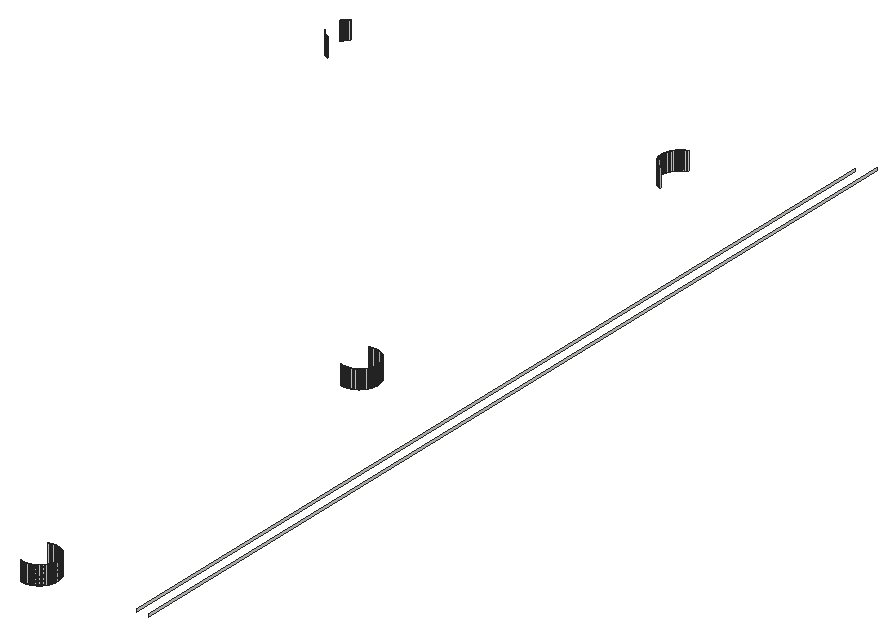
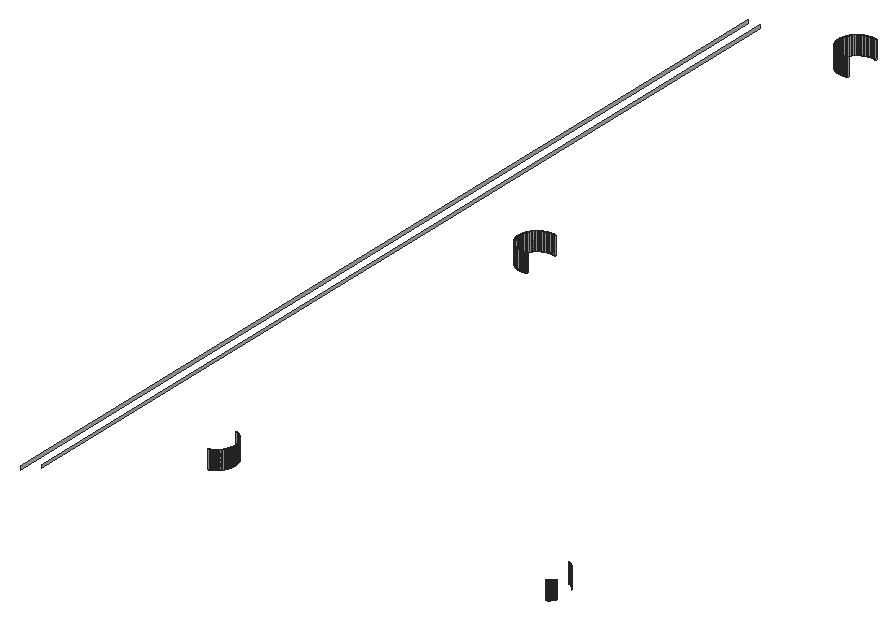
# SketchUp Ruby script. Lengths in inches.
U = 1.inch
M = Sketchup.active_model
def pt(a) = Geom::Point3d.new(a.map { |v| v * U })
def face(e, loops, mat)
  f = e.add_face(loops[0].map { |a| pt(a) })
  loops[1..].each { |l| e.add_face(l.map { |a| pt(a) }).erase! }
  f.material = f.back_material = mat if mat
  f
end
# faces: each face lists its corners as indices into pts; further lists are holes
def faces(e, pts, list, mat = nil) = list.each { |f| face(e, (f[0].is_a?(Array) ? f : [f]).map { |l| l.map { |i| pts[i] } }, mat) }
# xy, xz, yz: faces in a plane at the given z, y or x. An outline is a flat list of corners, or four numbers for a rectangle; further outlines are holes
def ring(l) = l.size == 4 ? [[l[0], l[1]], [l[2], l[1]], [l[2], l[3]], [l[0], l[3]]] : l.each_slice(2).to_a
def flat(e, list, mat, &to3) = list.each { |f| face(e, (f[0].is_a?(Array) ? f : [f]).map { |l| ring(l).map { |u, v| to3.(u, v) } }, mat) }
def xy(e, z, list, mat = nil) = flat(e, list, mat) { |x, y| [x, y, z] }
def xz(e, y, list, mat = nil) = flat(e, list, mat) { |x, z| [x, y, z] }
def yz(e, x, list, mat = nil) = flat(e, list, mat) { |y, z| [x, y, z] }
def lines(e, pts, list) = list.each { |a, b| e.add_line(pt(pts[a]), pt(pts[b])) }
# prism: a flat outline (further loops are holes) pulled along v
def prism(e, loops, v, mat = nil)
  f = face(e, loops, mat); d = Geom::Vector3d.new(v.map { |x| x * U })
  f.pushpull(f.normal.samedirection?(d) ? d.length : -d.length)
end
def box(e, o, s, mat = nil) = prism(e, [[o, [o[0] + s[0], o[1], o[2]], [o[0] + s[0], o[1] + s[1], o[2]], [o[0], o[1] + s[1], o[2]]]], [0, 0, s[2]], mat)
def at(x, y, z, deg = 0) = Geom::Transformation.translation(pt([x, y, z])) * Geom::Transformation.rotation(ORIGIN, Z_AXIS, deg.degrees)
def axes(o, x, y, z) = Geom::Transformation.new([*x, 0, *y, 0, *z, 0, *pt(o).to_a, 1])
def part(name) = M.definitions.add(name)
# library, detail: a bought-in or finely detailed component or shape, given as its bounding box
def library(name, o, s) = part(name).tap { |d| box(d.entities, o, s) }
def detail(e, o, s) = box(e.add_group.entities, o, s)
def put(e, d, t, mat = nil) = e.add_instance(d, t).tap { |i| i.material = mat if mat }
def group(e, t, mat = nil) = e.add_group.tap { |g| g.transformation = t; g.material = mat if mat }.entities
root = M.entities
xz(root,185,[[323.875,231,323.95,234],[323.95,231,324.03,234],[324.03,231,324.11,234]])
xz(root,185.01,[[323.72,231,323.8,234],[324.19,231,324.27,234]])
xz(root,190.99,[[323.73,231,323.81,234],[324.2,231,324.28,234]])
xz(root,191,[[323.89,231,323.97,234],[323.97,231,324.05,234],[324.05,231,324.125,234]])
xz(root,251,[[323.875,231,323.95,234],[323.95,231,324.03,234],[324.03,231,324.11,234]])
xz(root,251.01,[[323.72,231,323.8,234],[324.19,231,324.27,234]])
xz(root,256.99,[[323.73,231,323.81,234],[324.2,231,324.28,234]])
xz(root,257,[[323.89,231,323.97,234],[323.97,231,324.05,234],[324.05,231,324.125,234]])
yz(root,321,[[319.89,231,319.97,234],[319.97,231,320.05,234],[320.05,231,320.125,234]])
yz(root,321.01,[[319.73,231,319.81,234],[320.2,231,320.28,234]])
yz(root,326.99,[[187.72,231,187.8,234],[188.19,231,188.27,234],[253.72,231,253.8,234],[254.19,231,254.27,234]])
yz(root,327,[[187.875,231,187.95,234],[187.95,231,188.03,234],[188.03,231,188.11,234],[253.875,231,253.95,234],[253.95,231,254.03,234],
  [254.03,231,254.11,234]])
yz(root,340,[[188,231,336,231.5]])
yz(root,342,[[188,231,338,231.5]])
p = [[323.49,185.04,231],[323.41,185.06,231],[323.41,185.06,234],[323.49,185.04,234],[323.5625,185.03,231],[323.5625,185.03,234],
  [323.64,185.02,231],[323.64,185.02,234],[323.72,185.01,231],[323.72,185.01,234],[323.875,185,231],[323.8,185.01,231],
  [323.8,185.01,234],[323.875,185,234],[324.19,185.01,231],[324.11,185,231],[324.11,185,234],[324.19,185.01,234],
  [324.35,185.02,231],[324.27,185.01,231],[324.27,185.01,234],[324.35,185.02,234],[324.42,185.03,231],[324.42,185.03,234],
  [324.5,185.04,231],[324.5,185.04,234],[324.58,185.06,231],[324.58,185.06,234],[323.18,185.11,231],[323.1,185.14,231],
  [323.1,185.14,234],[323.18,185.11,234],[323.26,185.09,231],[323.26,185.09,234],[323.33,185.08,231],[323.33,185.08,234],
  [324.66,185.07,231],[324.66,185.07,234],[324.73,185.09,231],[324.73,185.09,234],[324.81,185.11,231],[324.81,185.11,234],
  [324.88,185.13,231],[324.88,185.13,234],[324.96,185.16,231],[324.96,185.16,234],[325.03,185.18,231],[325.03,185.18,234],
  [325.11,185.21,231],[325.11,185.21,234],[325.18,185.24,231],[325.18,185.24,234],[325.25,185.27,231],[325.25,185.27,234],
  [325.32,185.31,231],[325.32,185.31,234],[325.39,185.34,231],[325.39,185.34,234],[325.46,185.38,231],[325.46,185.38,234],
  [325.53,185.42,231],[325.53,185.42,234],[325.6,185.46,231],[325.6,185.46,234],[325.66,185.5,231],[325.66,185.5,234],
  [325.73,185.55,231],[325.73,185.55,234],[325.79,185.59,231],[325.79,185.59,234],[325.85,185.64,231],[325.85,185.64,234],
  [325.91,185.69,231],[325.91,185.69,234],[325.97,185.74,231],[325.97,185.74,234],[326.03,185.79,231],[326.03,185.79,234],
  [326.09,185.85,231],[326.09,185.85,234],[326.14,185.9,231],[326.14,185.9,234],[326.2,185.96,231],[326.2,185.96,234],
  [326.25,186.02,231],[326.25,186.02,234],[326.3,186.08,231],[326.3,186.08,234],[326.35,186.14,231],[326.35,186.14,234],
  [326.4,186.2,231],[326.4,186.2,234],[326.45,186.26,231],[326.45,186.26,234],[326.49,186.33,231],[326.49,186.33,234],
  [326.53,186.39,231],[326.53,186.39,234],[326.58,186.46,231],[326.58,186.46,234],[326.61,186.53,231],[326.61,186.53,234],
  [326.65,186.6,231],[326.65,186.6,234],[326.6875,186.67,231],[326.6875,186.67,234],[326.72,186.74,231],[326.72,186.74,234],
  [326.75,186.81,231],[326.75,186.81,234],[326.78,186.88,231],[326.78,186.88,234],[326.8125,186.96,231],[326.8125,186.96,234],
  [326.84,187.03,231],[326.84,187.03,234],[326.86,187.1,231],[326.86,187.1,234],[326.89,187.18,231],[326.89,187.18,234],
  [326.91,187.26,231],[326.91,187.26,234],[326.92,187.33,231],[326.92,187.33,234],[326.94,187.41,231],[326.94,187.41,234],
  [326.96,187.49,231],[326.96,187.49,234],[326.97,187.5625,231],[326.97,187.5625,234],[326.98,187.64,231],[326.98,187.64,234],
  [326.99,187.72,231],[326.99,187.72,234],[327,187.875,231],[326.99,187.8,231],[326.99,187.8,234],[327,187.875,234],
  [326.99,188.19,231],[327,188.11,231],[327,188.11,234],[326.99,188.19,234],[326.97,188.42,231],[326.98,188.35,231],
  [326.98,188.35,234],[326.97,188.42,234],[326.99,188.27,231],[326.99,188.27,234],[326.96,188.5,231],[326.96,188.5,234],
  [326.94,188.58,231],[326.94,188.58,234],[326.93,188.66,231],[326.93,188.66,234],[326.89,188.81,231],[326.91,188.73,231],
  [326.91,188.73,234],[326.89,188.81,234],[326.87,188.88,231],[326.87,188.88,234],[326.84,188.96,231],[326.84,188.96,234],
  [326.79,189.11,231],[326.82,189.03,231],[326.82,189.03,234],[326.79,189.11,234],[326.76,189.18,231],[326.76,189.18,234],
  [326.73,189.25,231],[326.73,189.25,234],[326.66,189.39,231],[326.69,189.32,231],[326.69,189.32,234],[326.66,189.39,234],
  [326.62,189.46,231],[326.62,189.46,234],[326.54,189.6,231],[326.58,189.53,231],[326.58,189.53,234],[326.54,189.6,234],
  [326.5,189.66,231],[326.5,189.66,234],[326.41,189.79,231],[326.45,189.73,231],[326.45,189.73,234],[326.41,189.79,234],
  [326.36,189.85,231],[326.36,189.85,234],[326.26,189.97,231],[326.31,189.91,231],[326.31,189.91,234],[326.26,189.97,234],
  [326.15,190.09,231],[326.21,190.03,231],[326.21,190.03,234],[326.15,190.09,234],[326.04,190.2,231],[326.1,190.14,231],
  [326.1,190.14,234],[326.04,190.2,234],[325.98,190.25,231],[325.98,190.25,234],[325.86,190.35,231],[325.92,190.3,231],
  [325.92,190.3,234],[325.86,190.35,234],[325.67,190.49,231],[325.74,190.45,231],[325.74,190.45,234],[325.67,190.49,234],
  [325.8,190.4,231],[325.8,190.4,234],[325.54,190.58,231],[325.61,190.53,231],[325.61,190.53,234],[325.54,190.58,234],
  [325.4,190.65,231],[325.47,190.61,231],[325.47,190.61,234],[325.4,190.65,234],[325.19,190.75,231],[325.26,190.72,231],
  [325.26,190.72,234],[325.19,190.75,234],[325.33,190.6875,231],[325.33,190.6875,234],[324.9,190.86,231],[324.97,190.84,231],
  [324.97,190.84,234],[324.9,190.86,234],[325.04,190.8125,231],[325.04,190.8125,234],[325.12,190.78,231],[325.12,190.78,234],
  [323.12,190.87,231],[323.19,190.89,231],[323.19,190.89,234],[323.12,190.87,234],[323.27,190.91,231],[323.27,190.91,234],
  [323.34,190.93,231],[323.34,190.93,234],[323.42,190.94,231],[323.42,190.94,234],[323.5,190.96,231],[323.5,190.96,234],
  [324.51,190.96,231],[324.59,190.94,231],[324.59,190.94,234],[324.51,190.96,234],[324.67,190.92,231],[324.67,190.92,234],
  [324.74,190.91,231],[324.74,190.91,234],[324.82,190.89,231],[324.82,190.89,234],[323.58,190.97,231],[323.58,190.97,234],
  [323.65,190.98,231],[323.65,190.98,234],[323.73,190.99,231],[323.73,190.99,234],[323.81,190.99,231],[323.89,191,231],
  [323.89,191,234],[323.81,190.99,234],[324.125,191,231],[324.2,190.99,231],[324.2,190.99,234],[324.125,191,234],
  [324.28,190.99,231],[324.36,190.98,231],[324.36,190.98,234],[324.28,190.99,234],[324.4375,190.97,231],[324.4375,190.97,234],
  [323.49,251.04,231],[323.41,251.06,231],[323.41,251.06,234],[323.49,251.04,234],[323.5625,251.03,231],[323.5625,251.03,234],
  [323.64,251.02,231],[323.64,251.02,234],[323.72,251.01,231],[323.72,251.01,234],[323.875,251,231],[323.8,251.01,231],
  [323.8,251.01,234],[323.875,251,234],[324.19,251.01,231],[324.11,251,231],[324.11,251,234],[324.19,251.01,234],
  [324.35,251.02,231],[324.27,251.01,231],[324.27,251.01,234],[324.35,251.02,234],[324.42,251.03,231],[324.42,251.03,234],
  [324.5,251.04,231],[324.5,251.04,234],[324.58,251.06,231],[324.58,251.06,234],[323.18,251.11,231],[323.1,251.14,231],
  [323.1,251.14,234],[323.18,251.11,234],[323.26,251.09,231],[323.26,251.09,234],[323.33,251.08,231],[323.33,251.08,234],
  [324.66,251.07,231],[324.66,251.07,234],[324.73,251.09,231],[324.73,251.09,234],[324.81,251.11,231],[324.81,251.11,234],
  [324.88,251.13,231],[324.88,251.13,234],[324.96,251.16,231],[324.96,251.16,234],[325.03,251.18,231],[325.03,251.18,234],
  [325.11,251.21,231],[325.11,251.21,234],[325.18,251.24,231],[325.18,251.24,234],[325.25,251.27,231],[325.25,251.27,234],
  [325.32,251.31,231],[325.32,251.31,234],[325.39,251.34,231],[325.39,251.34,234],[325.46,251.38,231],[325.46,251.38,234],
  [325.53,251.42,231],[325.53,251.42,234],[325.6,251.46,231],[325.6,251.46,234],[325.66,251.5,231],[325.66,251.5,234],
  [325.73,251.55,231],[325.73,251.55,234],[325.79,251.59,231],[325.79,251.59,234],[325.85,251.64,231],[325.85,251.64,234],
  [325.91,251.69,231],[325.91,251.69,234],[325.97,251.74,231],[325.97,251.74,234],[326.03,251.79,231],[326.03,251.79,234],
  [326.09,251.85,231],[326.09,251.85,234],[326.14,251.9,231],[326.14,251.9,234],[326.2,251.96,231],[326.2,251.96,234],
  [326.25,252.02,231],[326.25,252.02,234],[326.3,252.08,231],[326.3,252.08,234],[326.35,252.14,231],[326.35,252.14,234],
  [326.4,252.2,231],[326.4,252.2,234],[326.45,252.26,231],[326.45,252.26,234],[326.49,252.33,231],[326.49,252.33,234],
  [326.53,252.39,231],[326.53,252.39,234],[326.58,252.46,231],[326.58,252.46,234],[326.61,252.53,231],[326.61,252.53,234],
  [326.65,252.6,231],[326.65,252.6,234],[326.6875,252.67,231],[326.6875,252.67,234],[326.72,252.74,231],[326.72,252.74,234],
  [326.75,252.81,231],[326.75,252.81,234],[326.78,252.88,231],[326.78,252.88,234],[326.8125,252.96,231],[326.8125,252.96,234],
  [326.84,253.03,231],[326.84,253.03,234],[326.86,253.1,231],[326.86,253.1,234],[326.89,253.18,231],[326.89,253.18,234],
  [326.91,253.26,231],[326.91,253.26,234],[326.92,253.33,231],[326.92,253.33,234],[326.94,253.41,231],[326.94,253.41,234],
  [326.96,253.49,231],[326.96,253.49,234],[326.97,253.5625,231],[326.97,253.5625,234],[326.98,253.64,231],[326.98,253.64,234],
  [326.99,253.72,231],[326.99,253.72,234],[327,253.875,231],[326.99,253.8,231],[326.99,253.8,234],[327,253.875,234],
  [326.99,254.19,231],[327,254.11,231],[327,254.11,234],[326.99,254.19,234],[326.97,254.42,231],[326.98,254.35,231],
  [326.98,254.35,234],[326.97,254.42,234],[326.99,254.27,231],[326.99,254.27,234],[326.96,254.5,231],[326.96,254.5,234],
  [326.94,254.58,231],[326.94,254.58,234],[326.93,254.66,231],[326.93,254.66,234],[326.89,254.81,231],[326.91,254.73,231],
  [326.91,254.73,234],[326.89,254.81,234],[326.87,254.88,231],[326.87,254.88,234],[326.84,254.96,231],[326.84,254.96,234],
  [326.79,255.11,231],[326.82,255.03,231],[326.82,255.03,234],[326.79,255.11,234],[326.76,255.18,231],[326.76,255.18,234],
  [326.73,255.25,231],[326.73,255.25,234],[326.66,255.39,231],[326.69,255.32,231],[326.69,255.32,234],[326.66,255.39,234],
  [326.62,255.46,231],[326.62,255.46,234],[326.54,255.6,231],[326.58,255.53,231],[326.58,255.53,234],[326.54,255.6,234],
  [326.5,255.66,231],[326.5,255.66,234],[326.41,255.79,231],[326.45,255.73,231],[326.45,255.73,234],[326.41,255.79,234],
  [326.36,255.85,231],[326.36,255.85,234],[326.26,255.97,231],[326.31,255.91,231],[326.31,255.91,234],[326.26,255.97,234],
  [326.15,256.09,231],[326.21,256.03,231],[326.21,256.03,234],[326.15,256.09,234],[326.04,256.2,231],[326.1,256.14,231],
  [326.1,256.14,234],[326.04,256.2,234],[325.98,256.25,231],[325.98,256.25,234],[325.86,256.35,231],[325.92,256.3,231],
  [325.92,256.3,234],[325.86,256.35,234],[325.67,256.49,231],[325.74,256.45,231],[325.74,256.45,234],[325.67,256.49,234],
  [325.8,256.4,231],[325.8,256.4,234],[325.54,256.58,231],[325.61,256.53,231],[325.61,256.53,234],[325.54,256.58,234],
  [325.4,256.65,231],[325.47,256.61,231],[325.47,256.61,234],[325.4,256.65,234],[325.19,256.75,231],[325.26,256.72,231],
  [325.26,256.72,234],[325.19,256.75,234],[325.33,256.6875,231],[325.33,256.6875,234],[324.9,256.86,231],[324.97,256.84,231],
  [324.97,256.84,234],[324.9,256.86,234],[325.04,256.8125,231],[325.04,256.8125,234],[325.12,256.78,231],[325.12,256.78,234],
  [323.12,256.87,231],[323.19,256.89,231],[323.19,256.89,234],[323.12,256.87,234],[323.27,256.91,231],[323.27,256.91,234],
  [323.34,256.93,231],[323.34,256.93,234],[323.42,256.94,231],[323.42,256.94,234],[323.5,256.96,231],[323.5,256.96,234],
  [324.51,256.96,231],[324.59,256.94,231],[324.59,256.94,234],[324.51,256.96,234],[324.67,256.92,231],[324.67,256.92,234],
  [324.74,256.91,231],[324.74,256.91,234],[324.82,256.89,231],[324.82,256.89,234],[323.58,256.97,231],[323.58,256.97,234],
  [323.65,256.98,231],[323.65,256.98,234],[323.73,256.99,231],[323.73,256.99,234],[323.81,256.99,231],[323.89,257,231],
  [323.89,257,234],[323.81,256.99,234],[324.125,257,231],[324.2,256.99,231],[324.2,256.99,234],[324.125,257,234],
  [324.28,256.99,231],[324.36,256.98,231],[324.36,256.98,234],[324.28,256.99,234],[324.4375,256.97,231],[324.4375,256.97,234],
  [268.3,317.14,231],[268.23,317.16,231],[268.23,317.16,234],[268.3,317.14,234],[323.1,317.14,231],[323.03,317.16,231],
  [323.03,317.16,234],[323.1,317.14,234],[268.01,317.25,231],[267.9375,317.28,231],[267.9375,317.28,234],[268.01,317.25,234],
  [268.08,317.22,231],[268.08,317.22,234],[268.16,317.1875,231],[268.16,317.1875,234],[322.81,317.25,231],[322.74,317.28,231],
  [322.74,317.28,234],[322.81,317.25,234],[322.88,317.22,231],[322.88,317.22,234],[322.96,317.1875,231],[322.96,317.1875,234],
  [267.8,317.35,231],[267.73,317.39,231],[267.73,317.39,234],[267.8,317.35,234],[267.87,317.3125,231],[267.87,317.3125,234],
  [322.6,317.35,231],[322.53,317.39,231],[322.53,317.39,234],[322.6,317.35,234],[322.67,317.3125,231],[322.67,317.3125,234],
  [267.66,317.42,231],[267.59,317.47,231],[267.59,317.47,234],[267.66,317.42,234],[322.46,317.42,231],[322.39,317.47,231],
  [322.39,317.47,234],[322.46,317.42,234],[267.53,317.51,231],[267.46,317.55,231],[267.46,317.55,234],[267.53,317.51,234],
  [322.33,317.51,231],[322.26,317.55,231],[322.26,317.55,234],[322.33,317.51,234],[267.34,317.65,231],[267.28,317.7,231],
  [267.28,317.7,234],[267.34,317.65,234],[267.4,317.6,231],[267.4,317.6,234],[322.14,317.65,231],[322.08,317.7,231],
  [322.08,317.7,234],[322.14,317.65,234],[322.2,317.6,231],[322.2,317.6,234],[267.22,317.75,231],[267.16,317.8,231],
  [267.16,317.8,234],[267.22,317.75,234],[322.02,317.75,231],[321.96,317.8,231],[321.96,317.8,234],[322.02,317.75,234],
  [267.1,317.86,231],[267.1,317.86,234],[321.9,317.86,231],[321.9,317.86,234],[267.05,317.91,231],[266.99,317.97,231],
  [266.99,317.97,234],[267.05,317.91,234],[321.85,317.91,231],[321.79,317.97,231],[321.79,317.97,234],[321.85,317.91,234],
  [266.94,318.03,231],[266.89,318.09,231],[266.89,318.09,234],[266.94,318.03,234],[321.74,318.03,231],[321.69,318.09,231],
  [321.69,318.09,234],[321.74,318.03,234],[266.84,318.15,231],[266.79,318.21,231],[266.79,318.21,234],[266.84,318.15,234],
  [321.64,318.15,231],[321.59,318.21,231],[321.59,318.21,234],[321.64,318.15,234],[266.75,318.27,231],[266.75,318.27,234],
  [321.55,318.27,231],[321.55,318.27,234],[266.7,318.34,231],[266.66,318.4,231],[266.66,318.4,234],[266.7,318.34,234],
  [321.5,318.34,231],[321.46,318.4,231],[321.46,318.4,234],[321.5,318.34,234],[321.42,318.47,231],[321.42,318.47,234],
  [321.38,318.54,231],[321.34,318.61,231],[321.34,318.61,234],[321.38,318.54,234],[321.31,318.68,231],[321.31,318.68,234],
  [321.27,318.75,231],[321.24,318.82,231],[321.24,318.82,234],[321.27,318.75,234],[321.21,318.89,231],[321.21,318.89,234],
  [321.18,318.97,231],[321.18,318.97,234],[321.16,319.04,231],[321.13,319.12,231],[321.13,319.12,234],[321.16,319.04,234],
  [321.11,319.19,231],[321.11,319.19,234],[321.09,319.27,231],[321.09,319.27,234],[321.07,319.34,231],[321.06,319.42,231],
  [321.06,319.42,234],[321.07,319.34,234],[321.04,319.5,231],[321.04,319.5,234],[321.03,319.58,231],[321.03,319.58,234],
  [321.02,319.65,231],[321.02,319.65,234],[321.01,319.73,231],[321.01,319.73,234],[321.01,319.81,231],[321,319.89,231],
  [321,319.89,234],[321.01,319.81,234],[321,320.125,231],[321.01,320.2,231],[321.01,320.2,234],[321,320.125,234],
  [321.01,320.28,231],[321.02,320.36,231],[321.02,320.36,234],[321.01,320.28,234],[321.03,320.4375,231],[321.03,320.4375,234],
  [321.04,320.51,231],[321.04,320.51,234],[321.06,320.59,231],[321.06,320.59,234],[321.08,320.67,231],[321.08,320.67,234],
  [321.09,320.74,231],[321.09,320.74,234],[321.11,320.82,231],[321.11,320.82,234],[321.14,320.9,231],[321.14,320.9,234],
  [321.16,320.97,231],[321.16,320.97,234],[321.1875,321.04,231],[321.1875,321.04,234],[321.22,321.12,231],[321.22,321.12,234],
  [321.25,321.19,231],[321.25,321.19,234],[321.28,321.26,231],[321.28,321.26,234],[321.3125,321.33,231],[321.3125,321.33,234],
  [321.35,321.4,231],[321.35,321.4,234],[321.39,321.47,231],[321.39,321.47,234],[321.42,321.54,231],[321.42,321.54,234],
  [321.47,321.61,231],[321.47,321.61,234],[266.67,321.61,231],[266.71,321.67,231],[266.71,321.67,234],[266.67,321.61,234],
  [321.51,321.67,231],[321.51,321.67,234],[266.75,321.74,231],[266.75,321.74,234],[266.8,321.8,231],[266.8,321.8,234],
  [321.55,321.74,231],[321.55,321.74,234],[321.6,321.8,231],[321.6,321.8,234],[266.85,321.86,231],[266.85,321.86,234],
  [321.65,321.86,231],[321.65,321.86,234],[266.9,321.92,231],[266.9,321.92,234],[266.95,321.98,231],[266.95,321.98,234],
  [321.7,321.92,231],[321.7,321.92,234],[321.75,321.98,231],[321.75,321.98,234],[267,322.04,231],[267,322.04,234],
  [267.06,322.1,231],[267.06,322.1,234],[321.8,322.04,231],[321.8,322.04,234],[321.86,322.1,231],[321.86,322.1,234],
  [267.11,322.15,231],[267.11,322.15,234],[321.91,322.15,231],[321.91,322.15,234],[267.17,322.21,231],[267.17,322.21,234],
  [267.23,322.26,231],[267.23,322.26,234],[321.97,322.21,231],[321.97,322.21,234],[322.03,322.26,231],[322.03,322.26,234],
  [267.29,322.31,231],[267.29,322.31,234],[267.35,322.36,231],[267.35,322.36,234],[322.09,322.31,231],[322.09,322.31,234],
  [322.15,322.36,231],[322.15,322.36,234],[267.41,322.41,231],[267.41,322.41,234],[267.47,322.45,231],[267.47,322.45,234],
  [322.21,322.41,231],[322.21,322.41,234],[322.27,322.45,231],[322.27,322.45,234],[267.54,322.5,231],[267.54,322.5,234],
  [267.6,322.54,231],[267.6,322.54,234],[267.67,322.58,231],[267.67,322.58,234],[322.34,322.5,231],[322.34,322.5,234],
  [322.4,322.54,231],[322.4,322.54,234],[322.47,322.58,231],[322.47,322.58,234],[322.54,322.62,231],[322.54,322.62,234],
  [322.61,322.66,231],[322.61,322.66,234],[322.68,322.69,231],[322.68,322.69,234],[322.75,322.73,231],[322.75,322.73,234],
  [322.82,322.76,231],[322.82,322.76,234],[322.89,322.79,231],[322.89,322.79,234],[322.97,322.82,231],[322.97,322.82,234],
  [323.04,322.84,231],[323.04,322.84,234],[323.12,322.87,231],[323.12,322.87,234]]
faces(root,p,[[0,1,2,3],[4,0,3,5],[6,4,5,7],[8,6,7,9],[10,11,12,13],[14,15,16,17],[18,19,20,21],[22,18,21,23],
  [24,22,23,25],[26,24,25,27],[28,29,30,31],[32,28,31,33],[34,32,33,35],[1,34,35,2],[36,26,27,37],[38,36,37,39],
  [40,38,39,41],[42,40,41,43],[44,42,43,45],[46,44,45,47],[48,46,47,49],[50,48,49,51],[52,50,51,53],[54,52,53,55],
  [56,54,55,57],[58,56,57,59],[60,58,59,61],[62,60,61,63],[64,62,63,65],[66,64,65,67],[68,66,67,69],[70,68,69,71],
  [72,70,71,73],[74,72,73,75],[76,74,75,77],[78,76,77,79],[80,78,79,81],[82,80,81,83],[84,82,83,85],[86,84,85,87],
  [88,86,87,89],[90,88,89,91],[92,90,91,93],[94,92,93,95],[96,94,95,97],[98,96,97,99],[100,98,99,101],[102,100,101,103],
  [104,102,103,105],[106,104,105,107],[108,106,107,109],[110,108,109,111],[112,110,111,113],[114,112,113,115],[116,114,115,117],[118,116,117,119],
  [120,118,119,121],[122,120,121,123],[124,122,123,125],[126,124,125,127],[128,126,127,129],[130,128,129,131],[132,130,131,133],[134,135,136,137],
  [138,139,140,141],[142,143,144,145],[143,146,147,144],[148,142,145,149],[150,148,149,151],[152,150,151,153],[154,155,156,157],[155,152,153,156],
  [158,154,157,159],[160,158,159,161],[162,163,164,165],[163,160,161,164],[166,162,165,167],[168,166,167,169],[170,171,172,173],[171,168,169,172],
  [174,170,173,175],[176,177,178,179],[177,174,175,178],[180,176,179,181],[182,183,184,185],[183,180,181,184],[186,182,185,187],[188,189,190,191],
  [189,186,187,190],[192,193,194,195],[193,188,191,194],[196,197,198,199],[197,192,195,198],[200,196,199,201],[202,203,204,205],[203,200,201,204],
  [206,207,208,209],[207,210,211,208],[210,202,205,211],[212,213,214,215],[213,206,209,214],[216,217,218,219],[217,212,215,218],[220,221,222,223],
  [221,224,225,222],[224,216,219,225],[226,227,228,229],[227,230,231,228],[230,232,233,231],[232,220,223,233],[234,235,236,237],[235,238,239,236],
  [238,240,241,239],[240,242,243,241],[242,244,245,243],[246,247,248,249],[247,250,251,248],[250,252,253,251],[252,254,255,253],[254,226,229,255],
  [244,256,257,245],[256,258,259,257],[258,260,261,259],[262,263,264,265],[266,267,268,269],[270,271,272,273],[271,274,275,272],[274,246,249,275],
  [276,277,278,279],[280,276,279,281],[282,280,281,283],[284,282,283,285],[286,287,288,289],[290,291,292,293],[294,295,296,297],[298,294,297,299],
  [300,298,299,301],[302,300,301,303],[304,305,306,307],[308,304,307,309],[310,308,309,311],[277,310,311,278],[312,302,303,313],[314,312,313,315],
  [316,314,315,317],[318,316,317,319],[320,318,319,321],[322,320,321,323],[324,322,323,325],[326,324,325,327],[328,326,327,329],[330,328,329,331],
  [332,330,331,333],[334,332,333,335],[336,334,335,337],[338,336,337,339],[340,338,339,341],[342,340,341,343],[344,342,343,345],[346,344,345,347],
  [348,346,347,349],[350,348,349,351],[352,350,351,353],[354,352,353,355],[356,354,355,357],[358,356,357,359],[360,358,359,361],[362,360,361,363],
  [364,362,363,365],[366,364,365,367],[368,366,367,369],[370,368,369,371],[372,370,371,373],[374,372,373,375],[376,374,375,377],[378,376,377,379],
  [380,378,379,381],[382,380,381,383],[384,382,383,385],[386,384,385,387],[388,386,387,389],[390,388,389,391],[392,390,391,393],[394,392,393,395],
  [396,394,395,397],[398,396,397,399],[400,398,399,401],[402,400,401,403],[404,402,403,405],[406,404,405,407],[408,406,407,409],[410,411,412,413],
  [414,415,416,417],[418,419,420,421],[419,422,423,420],[424,418,421,425],[426,424,425,427],[428,426,427,429],[430,431,432,433],[431,428,429,432],
  [434,430,433,435],[436,434,435,437],[438,439,440,441],[439,436,437,440],[442,438,441,443],[444,442,443,445],[446,447,448,449],[447,444,445,448],
  [450,446,449,451],[452,453,454,455],[453,450,451,454],[456,452,455,457],[458,459,460,461],[459,456,457,460],[462,458,461,463],[464,465,466,467],
  [465,462,463,466],[468,469,470,471],[469,464,467,470],[472,473,474,475],[473,468,471,474],[476,472,475,477],[478,479,480,481],[479,476,477,480],
  [482,483,484,485],[483,486,487,484],[486,478,481,487],[488,489,490,491],[489,482,485,490],[492,493,494,495],[493,488,491,494],[496,497,498,499],
  [497,500,501,498],[500,492,495,501],[502,503,504,505],[503,506,507,504],[506,508,509,507],[508,496,499,509],[510,511,512,513],[511,514,515,512],
  [514,516,517,515],[516,518,519,517],[518,520,521,519],[522,523,524,525],[523,526,527,524],[526,528,529,527],[528,530,531,529],[530,502,505,531],
  [520,532,533,521],[532,534,535,533],[534,536,537,535],[538,539,540,541],[542,543,544,545],[546,547,548,549],[547,550,551,548],[550,522,525,551],
  [552,553,554,555],[556,557,558,559],[560,561,562,563],[564,560,563,565],[566,564,565,567],[553,566,567,554],[568,569,570,571],[572,568,571,573],
  [574,572,573,575],[557,574,575,558],[576,577,578,579],[580,576,579,581],[561,580,581,562],[582,583,584,585],[586,582,585,587],[569,586,587,570],
  [588,589,590,591],[577,588,591,578],[592,593,594,595],[583,592,595,584],[596,597,598,599],[589,596,599,590],[600,601,602,603],[593,600,603,594],
  [604,605,606,607],[608,604,607,609],[597,608,609,598],[610,611,612,613],[614,610,613,615],[601,614,615,602],[616,617,618,619],[605,616,619,606],
  [620,621,622,623],[611,620,623,612],[617,624,625,618],[621,626,627,622],[628,629,630,631],[624,628,631,625],[632,633,634,635],[626,632,635,627],
  [636,637,638,639],[629,636,639,630],[640,641,642,643],[633,640,643,634],[644,645,646,647],[637,644,647,638],[648,649,650,651],[641,648,651,642],
  [645,652,653,646],[649,654,655,650],[656,657,658,659],[652,656,659,653],[660,661,662,663],[654,660,663,655],[661,664,665,662],[666,667,668,669],
  [664,666,669,665],[667,670,671,668],[672,673,674,675],[670,672,675,671],[673,676,677,674],[676,678,679,677],[680,681,682,683],[678,680,683,679],
  [681,684,685,682],[684,686,687,685],[688,689,690,691],[686,688,691,687],[689,692,693,690],[692,694,695,693],[694,696,697,695],[696,698,699,697],
  [700,701,702,703],[704,705,706,707],[708,709,710,711],[709,712,713,710],[712,714,715,713],[714,716,717,715],[716,718,719,717],[718,720,721,719],
  [720,722,723,721],[722,724,725,723],[724,726,727,725],[726,728,729,727],[728,730,731,729],[730,732,733,731],[732,734,735,733],[734,736,737,735],
  [736,738,739,737],[738,740,741,739],[740,742,743,741],[742,744,745,743],[746,747,748,749],[744,750,751,745],[747,752,753,748],[752,754,755,753],
  [750,756,757,751],[756,758,759,757],[754,760,761,755],[758,762,763,759],[760,764,765,761],[764,766,767,765],[762,768,769,763],[768,770,771,769],
  [766,772,773,767],[772,774,775,773],[770,776,777,771],[776,778,779,777],[774,780,781,775],[778,782,783,779],[780,784,785,781],[784,786,787,785],
  [782,788,789,783],[788,790,791,789],[786,792,793,787],[792,794,795,793],[790,796,797,791],[796,798,799,797],[794,800,801,795],[800,802,803,801],
  [798,804,805,799],[804,806,807,805],[802,808,809,803],[808,810,811,809],[810,812,813,811],[806,814,815,807],[814,816,817,815],[816,818,819,817],
  [818,820,821,819],[820,822,823,821],[822,824,825,823],[824,826,827,825],[826,828,829,827],[828,830,831,829],[830,832,833,831],[832,834,835,833],
  [834,836,837,835]])
